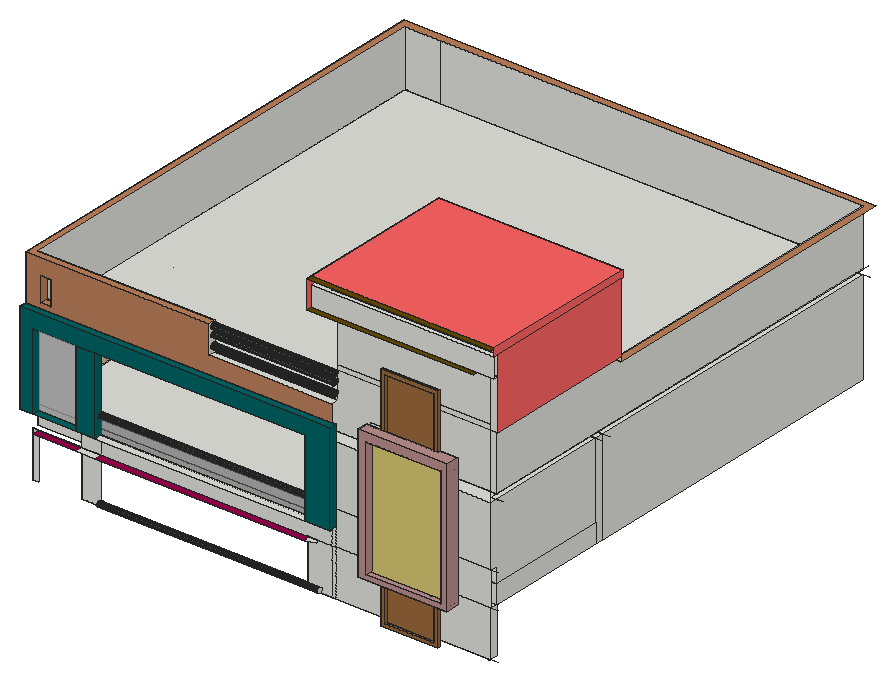
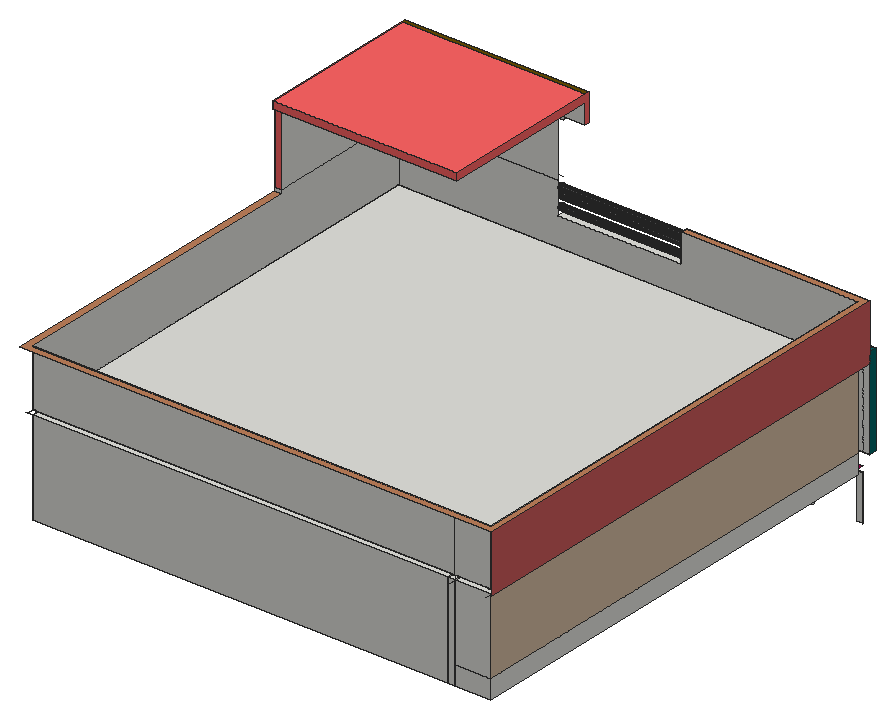
# SketchUp Ruby script. Lengths in inches.
U = 1.inch
M = Sketchup.active_model
def pt(a) = Geom::Point3d.new(a.map { |v| v * U })
def face(e, loops, mat)
  f = e.add_face(loops[0].map { |a| pt(a) })
  loops[1..].each { |l| e.add_face(l.map { |a| pt(a) }).erase! }
  f.material = f.back_material = mat if mat
  f
end
# faces: each face lists its corners as indices into pts; further lists are holes
def faces(e, pts, list, mat = nil) = list.each { |f| face(e, (f[0].is_a?(Array) ? f : [f]).map { |l| l.map { |i| pts[i] } }, mat) }
# xy, xz, yz: faces in a plane at the given z, y or x. An outline is a flat list of corners, or four numbers for a rectangle; further outlines are holes
def ring(l) = l.size == 4 ? [[l[0], l[1]], [l[2], l[1]], [l[2], l[3]], [l[0], l[3]]] : l.each_slice(2).to_a
def flat(e, list, mat, &to3) = list.each { |f| face(e, (f[0].is_a?(Array) ? f : [f]).map { |l| ring(l).map { |u, v| to3.(u, v) } }, mat) }
def xy(e, z, list, mat = nil) = flat(e, list, mat) { |x, y| [x, y, z] }
def xz(e, y, list, mat = nil) = flat(e, list, mat) { |x, z| [x, y, z] }
def yz(e, x, list, mat = nil) = flat(e, list, mat) { |y, z| [x, y, z] }
def lines(e, pts, list) = list.each { |a, b| e.add_line(pt(pts[a]), pt(pts[b])) }
# prism: a flat outline (further loops are holes) pulled along v
def prism(e, loops, v, mat = nil)
  f = face(e, loops, mat); d = Geom::Vector3d.new(v.map { |x| x * U })
  f.pushpull(f.normal.samedirection?(d) ? d.length : -d.length)
end
def box(e, o, s, mat = nil) = prism(e, [[o, [o[0] + s[0], o[1], o[2]], [o[0] + s[0], o[1] + s[1], o[2]], [o[0], o[1] + s[1], o[2]]]], [0, 0, s[2]], mat)
def at(x, y, z, deg = 0) = Geom::Transformation.translation(pt([x, y, z])) * Geom::Transformation.rotation(ORIGIN, Z_AXIS, deg.degrees)
def axes(o, x, y, z) = Geom::Transformation.new([*x, 0, *y, 0, *z, 0, *pt(o).to_a, 1])
def part(name) = M.definitions.add(name)
# library, detail: a bought-in or finely detailed component or shape, given as its bounding box
def library(name, o, s) = part(name).tap { |d| box(d.entities, o, s) }
def detail(e, o, s) = box(e.add_group.entities, o, s)
def put(e, d, t, mat = nil) = e.add_instance(d, t).tap { |i| i.material = mat if mat }
def group(e, t, mat = nil) = e.add_group.tap { |g| g.transformation = t; g.material = mat if mat }.entities
root = M.entities
M.materials.add("[0017_IndianRed]").color = [205, 92, 92]
M.materials.add("[0059_DarkOliveGreen]").color = [85, 107, 47]
M.materials.add("[0119_RosyBrown]").color = [188, 143, 143]
M.materials.add("[Color A03]").color = [255, 101, 101]
M.materials.add("[Color C04]").color = [255, 153, 50]
M.materials.add("[Color D08]").color = [102, 76, 0]
M.materials.add("[Color H08]").color = [0, 102, 102]
M.materials.add("[Color L11]").color = [153, 0, 76]
M.materials.add("[Color M05]").color = [114, 114, 114]
M.materials.add("[Color M06]").color = [86, 86, 86]
M.materials.add("[Formica Laminate Light]").color = [213, 189, 164]
M.materials.add("[Mirror 02]").color = [229, 229, 229]
M.materials.add("[Translucent Glass Gray]").color = [128, 128, 128]
M.materials["[Translucent Glass Gray]"].alpha = 0.5
M.materials.add("[Translucent Resin Crush Gray]").color = [184, 184, 184]
M.materials["[Translucent Resin Crush Gray]"].alpha = 0.8
M.materials.add("[Wood Bamboo]").color = [177, 105, 43]
M.materials.add("[Wood Board Cork]").color = [215, 201, 115]
M.materials.add("[Wood Floor]").color = [155, 105, 61]
M.materials.add("[Wood Veneer 02]").color = [190, 128, 91]
xy(root,177.05,[[623.84,156.04,695.78,159.04]],"[Wood Floor]")
xy(root,181.3125,[[236.6,165.04,523.3,165.04,523.75,165.23,236.6875,165.23],[523.3,165.04,756.04,165.04,756.04,165.23,523.75,165.23]])
xy(root,181.49,[[628.28,156.04,691.34,159.04]],"[Wood Floor]")
xy(root,182.0625,[[236.6875,165.23,756.04,165.23,756.04,174.04,241.08,174.04]])
xy(root,204,[[441.07,324.28,448.45,324.28,448.45,328.59,466.45,328.59,466.45,331.59,430.45,331.59,430.45,328.59,441.07,328.59]])
xy(root,212.33,[[533.78,326.59,672.97,328.59],[533.78,328.59,672.97,331.59]])
xy(root,215.33,[[530.78,328.59,675.97,331.59]])
xy(root,232.57,[[605.59,142.54,605.59,156.04,695.78,156.04,695.78,159.04,718.71,159.04,718.71,142.54]],"[0119_RosyBrown]")
xy(root,237.91,[[614.97,150.6,615.87,153.04],[615.87,150.6,628.28,153.04],[628.28,150.6,691.34,153.04],[691.34,150.6,695.78,153.04],[695.78,150.6,710.3125,153.04],
  [614.97,153.04,615.87,156.04],[615.87,153.04,628.28,156.04],[628.28,153.04,691.34,156.04],[691.34,153.04,695.78,156.04],[695.78,153.04,710.3125,156.04],
  [628.28,156.04,691.34,159.04],[695.78,156.04,710.3125,159.04],[616.375,159.04,623.84,159.85]])
xy(root,237.91,[[615.87,142.54,710.3125,150.6]],"[0119_RosyBrown]")
xy(root,240,[[236.6,156.04,260.92,165.04],[527.08,156.04,538.15,160.69,536.32,165.04,523.3,165.04],[174.04,165.04,174.04,165.23,236.6875,165.23,241.08,174.04,756.04,174.04,756.04,165.04,536.32,165.04,534.36,169.69,523.3,165.04],[523.3,165.04,534.36,169.69,536.32,165.04],[174.04,174.04,185.29,756.04],
  [185.29,174.04,185.29,756.04,219.49,756.04,219.49,331.59,295.38,331.59,295.38,328.59,311.1,328.59,311.1,325.59,331.38,325.59,331.38,331.59,756.04,331.59,756.04,174.04],[311.1,325.59,331.38,328.59],[295.38,328.59,331.38,331.59],[219.49,331.59,219.49,756.04,229.13,756.04,229.13,342.77,756.04,342.77,756.04,331.59],[229.13,342.77,756.04,756.04]])
xy(root,240,[[181.38,156.04,236.6,165.04],[260.92,156.04,260.92,165.04,523.3,165.04,527.08,156.04]],"[Color L11]")
xy(root,242.39,[[313.49,325.59,328.99,328.59]])
xy(root,246.83,[[355.12,328.59,402.92,331.59]])
xy(root,252.33,[[360.61,328.59,397.43,331.59]])
xy(root,255.01,[[467.84,328.59,560.59,331.59]])
xy(root,260.13,[[472.97,328.59,555.47,331.59]])
xy(root,262.875,[[165.04,156.04,174.04,165.04],[174.04,156.04,181.38,165.04],[236.6,156.04,260.92,158.48],[260.92,156.04,527.08,165.04],[527.08,156.04,558.79,165.04],
  [558.79,156.04,559.05,165.04],[236.6,158.48,260.92,160.54]])
xy(root,262.875,[[181.38,156.04,236.6,165.04]],"[Color H08]")
xy(root,263.8125,[[174.04,174.04,756.04,174.04,756.04,331.59,331.38,331.59,331.38,325.59,311.1,325.59,311.1,328.59,295.38,328.59,295.38,331.59,219.49,331.59,219.49,756.04,174.04,756.04]])
xy(root,279.61,[[313.49,325.59,328.99,328.59]],"[Wood Bamboo]")
xy(root,282,[[311.1,325.59,331.38,328.59]],"[Wood Bamboo]")
xy(root,283.3125,[[236.6,165.04,756.04,165.04,756.04,174.04,246.18,174.04]])
xy(root,323.58,[[360.61,328.59,397.43,331.59]])
xy(root,324,[[295.38,328.59,331.38,331.59]],"[Wood Bamboo]")
xy(root,327.13,[[472.97,328.59,555.47,331.59]])
xy(root,329.08,[[355.12,328.59,402.92,331.59]])
xy(root,332.25,[[467.84,328.59,560.59,331.59]])
xy(root,360,[[236.6,156.04,260.92,160.54],[236.6,160.54,260.92,165.04],[236.6,165.04,246.18,174.04,174.04,174.04,174.04,756.04,219.49,756.04,219.49,331.59,756.04,331.59,756.04,165.04],[219.49,331.59,219.49,756.04,229.13,756.04,229.13,342.77,756.04,342.77,756.04,331.59],[229.13,342.77,756.04,756.04]])
xy(root,360,[[181.38,156.04,236.6,165.04],[260.92,156.04,527.08,165.04]],"[Color H08]")
xy(root,365.75,[[755.73,174.04,756.04,756.04]])
xy(root,366,[[174.04,174.04,756.04,756.04]])
xy(root,379.73,[[165.04,156.04,558.79,165.04]],"[Color H08]")
xy(root,386.57,[[184.31,165.04,197.75,174.04]],"[Wood Veneer 02]")
xy(root,389.91,[[605.43,142.54,605.59,152.54],[614.97,150.6,615.87,152.54],[615.87,150.6,628.28,152.54],[628.28,150.6,691.34,152.54],[691.34,150.6,695.78,152.54],
  [695.78,150.6,710.3125,152.54],[605.43,152.54,605.59,153.04],[605.59,152.54,607.89,153.04],[614.97,152.54,615.87,153.04],[615.87,152.54,628.28,152.54,628.28,156.04,614.97,156.04,614.97,153.04,615.87,153.04],
  [628.28,152.54,691.34,156.04],[691.34,152.54,695.78,156.04],[695.78,152.54,710.3125,156.04],[628.28,156.04,691.34,159.04],[695.78,156.04,710.3125,159.04],
  [616.375,159.04,623.84,159.85]])
xy(root,389.91,[[615.87,142.54,710.3125,150.6]],"[0119_RosyBrown]")
xy(root,400.38,[[605.43,142.54,718.71,142.54,718.71,159.04,695.78,159.04,695.78,156.04,605.59,156.04,605.59,153.04,605.43,153.04]],"[0119_RosyBrown]")
xy(root,401.875,[[398.38,165.04,554.6,174.04]])
xy(root,417.76,[[184.31,165.04,197.75,174.04]])
xy(root,437.75,[[165.04,165.04,398.38,165.04,398.38,174.04,174.04,174.04,174.04,756.04,756.04,756.04,756.04,360.73,765.04,360.73,765.04,765.04,165.04,765.04]],"[Wood Veneer 02]")
xy(root,464.8,[[628.28,156.04,691.34,159.04]])
xy(root,469.24,[[623.84,156.04,695.78,159.04]],"[Wood Floor]")
xy(root,506.1875,[[554.6,159.04,755.73,165.04],[755.73,159.04,765.04,165.04]])
xy(root,506.1875,[[531.67,153.04,743.6,159.04]],"[Color D08]")
xy(root,531.66,[[531.67,159.04,765.04,362.6]])
xy(root,541.25,[[531.67,159.04,765.04,362.6]],"[Color A03]")
xy(root,541.25,[[531.67,153.04,765.04,159.04]],"[Color D08]")
xz(root,142.54,[[[605.59,232.57,718.71,232.57,718.71,400.38,605.43,400.38,605.43,389.91,605.59,389.91],[615.87,237.91,710.3125,389.91]]],"[0119_RosyBrown]")
xz(root,150.6,[[614.97,237.91,710.3125,389.91]],"[Wood Board Cork]")
xz(root,153.04,[[605.43,389.91,605.59,400.38]])
xz(root,156.04,[[605.59,232.57,606.34,400.38],[606.34,232.57,606.34,400.38,607.89,400.38,607.89,389.91,607.9,389.91,607.9,232.57],[607.9,232.57,607.9,389.91,614.97,389.91,614.97,237.91,623.84,237.91,623.84,232.57],[623.84,232.57,628.28,237.91],[628.28,232.57,691.34,237.91],
  [614.97,237.91,615.87,389.91],[615.87,237.91,623.84,389.91],[623.84,237.91,628.28,389.91],[691.34,237.91,695.78,389.91],[695.78,237.91,710.3125,389.91],
  [607.89,389.91,607.9,400.38],[607.9,389.91,615.87,400.38],[615.87,389.91,623.84,400.38],[623.84,389.91,628.28,400.38],[628.28,389.91,691.34,400.38],
  [691.34,389.91,695.78,400.38]])
xz(root,156.04,[[165.04,262.875,181.38,262.875,181.38,360,527.08,360,527.08,262.875,558.79,262.875,558.79,379.73,165.04,379.73],[236.6,262.875,260.92,360]],"[Color H08]")
xz(root,156.04,[[623.84,177.05,695.78,177.05,695.78,232.57,691.34,232.57,691.34,181.49,628.28,181.49,628.28,232.57,623.84,232.57],[623.84,400.38,628.28,400.38,628.28,464.8,691.34,464.8,691.34,400.38,695.78,400.38,695.78,469.24,623.84,469.24]],"[Wood Floor]")
xz(root,159.04,[[623.84,177.05,623.84,232.57,628.28,232.57,628.28,181.49,691.34,181.49,691.34,232.57,695.78,232.57,695.78,177.05],[623.84,232.57,628.28,237.91],[691.34,232.57,695.78,237.91],[695.78,232.57,695.78,237.91,710.3125,237.91,710.3125,389.91,695.78,389.91,695.78,400.38,718.71,400.38,718.71,232.57],[616.375,237.91,623.84,389.91],
  [623.84,237.91,628.28,389.91],[628.28,237.91,691.34,389.91],[691.34,237.91,695.78,389.91],[695.78,237.91,710.3125,389.91],[623.84,389.91,628.28,400.38],
  [691.34,389.91,695.78,400.38],[623.84,400.38,623.84,469.24,695.78,469.24,695.78,400.38,691.34,400.38,691.34,464.8,628.28,464.8,628.28,400.38],[531.67,506.1875,765.04,531.66]])
xz(root,159.04,[[628.28,181.49,691.34,237.91],[628.28,389.91,691.34,464.8]],"[Wood Floor]")
xz(root,159.85,[[607.89,232.57,607.89,400.38,623.84,400.38,623.84,389.91,616.375,389.91,616.375,237.91,623.84,237.91,623.84,232.57]])
xz(root,165.04,[[174.04,181.3125,181.38,240],[236.6,181.3125,260.92,240],[523.3,181.3125,554.6,240],[554.6,181.3125,559.05,240],[559.05,181.3125,755.73,240],
  [755.73,181.3125,756.04,240],[236.6,240,260.92,262.875],[260.92,240,554.6,262.875],[554.6,240,559.05,262.875],[559.05,240,559.05,262.875,558.79,262.875,558.79,283.3125,755.73,283.3125,755.73,240],
  [165.04,262.875,165.04,379.73,554.6,379.73,554.6,360,174.04,360,174.04,262.875],[174.04,262.875,181.38,360],[236.6,262.875,260.92,283.3125],[527.08,262.875,554.6,283.3125],[554.6,262.875,558.79,283.3125],
  [236.6,283.3125,260.92,360],[527.08,283.3125,527.08,284.67,537.23,284.67,537.23,288.35,527.08,288.35,527.08,360,554.6,360,554.6,283.3125],[554.6,283.3125,558.79,360],[558.79,283.3125,755.73,360],[755.73,283.3125,756.04,360],
  [260.92,284.67,527.08,288.35],[527.08,284.67,537.23,288.35],[554.6,360,558.79,379.73],[755.73,442.375,765.04,506.1875],[554.6,506.1875,755.73,531],
  [755.73,506.1875,765.04,531],[554.6,531,755.73,533.3125],[755.73,531,765.04,533.3125]])
xz(root,165.04,[[260.92,262.875,527.08,283.3125]],"[Translucent Glass Gray]")
xz(root,165.04,[[181.38,262.875,236.6,360]],"[Translucent Resin Crush Gray]")
xz(root,165.04,[[[165.04,379.73,554.6,379.73,554.6,401.875,398.38,401.875,398.38,437.75,165.04,437.75],[184.31,386.57,197.75,417.76]]],"[Wood Veneer 02]")
xz(root,165.23,[[236.6875,181.3125,523.75,182.0625],[523.75,181.3125,756.04,182.0625]])
xz(root,174.04,[[174.04,240,756.04,263.8125],[174.04,365.75,756.04,366],[[174.04,366,174.04,437.75,398.38,437.75,398.38,401.875,554.6,401.875,554.6,442.375,756.04,442.375,756.04,366],[184.31,386.57,197.75,417.76]],[554.6,442.375,756.04,531],[554.6,531,756.04,533.3125]])
xz(root,174.04,[[174.04,263.8125,174.04,360,246.18,360,246.18,283.3125,756.04,283.3125,756.04,263.8125]],"[Mirror 02]")
xz(root,325.59,[[311.1,240,331.38,240,331.38,263.8125,328.99,263.8125,328.99,242.39,313.49,242.39,313.49,263.8125,311.1,263.8125],[313.49,242.39,328.99,263.8125]])
xz(root,325.59,[[311.1,263.8125,313.49,263.8125,313.49,279.61,328.99,279.61,328.99,263.8125,331.38,263.8125,331.38,282,311.1,282]],"[Wood Bamboo]")
xz(root,328.59,[[295.38,240,311.1,263.8125],[[311.1,240,331.38,282],[313.49,242.39,328.99,279.61]]])
xz(root,328.59,[[[355.12,246.83,402.92,329.08],[360.61,252.33,397.43,323.58]],[[467.84,255.01,560.59,332.25],[472.97,260.13,555.47,327.13]]],"[Color C04]")
xz(root,328.59,[[313.49,242.39,328.99,279.61],[[295.38,263.8125,311.1,263.8125,311.1,282,331.38,282,331.38,324,295.38,324],[308.81,285.54,301.94,285.86,298.78,291.97,302.49,297.76,309.36,297.4375,312.52,291.33]],[308.81,285.54,312.52,291.33,309.36,297.4375,302.49,297.76,298.78,291.97,301.94,285.86]],"[Wood Bamboo]")
xz(root,331.59,[[219.49,240,295.38,263.8125],[295.38,240,331.38,324],[331.38,240,331.38,263.8125,355.12,263.8125,355.12,246.83,402.92,246.83,402.92,263.8125,467.84,263.8125,467.84,255.01,560.59,255.01,560.59,263.8125,756.04,263.8125,756.04,240],[355.12,246.83,355.12,263.8125,360.61,263.8125,360.61,252.33,397.43,252.33,397.43,263.8125,402.92,263.8125,402.92,246.83],[360.61,252.33,397.43,263.8125],
  [467.84,255.01,467.84,263.8125,472.97,263.8125,472.97,260.13,555.47,260.13,555.47,263.8125,560.59,263.8125,560.59,255.01],[472.97,260.13,555.47,263.8125],[355.12,263.8125,355.12,329.08,402.92,329.08,402.92,263.8125,397.43,263.8125,397.43,323.58,360.61,323.58,360.61,263.8125],[467.84,263.8125,467.84,332.25,560.59,332.25,560.59,263.8125,555.47,263.8125,555.47,327.13,472.97,327.13,472.97,263.8125]])
xz(root,331.59,[[219.49,263.8125,295.38,263.8125,295.38,324,331.38,324,331.38,263.8125,355.12,263.8125,355.12,329.08,402.92,329.08,402.92,263.8125,467.84,263.8125,467.84,332.25,560.59,332.25,560.59,263.8125,756.04,263.8125,756.04,360,219.49,360]],"[Formica Laminate Light]")
xz(root,331.59,[[360.61,263.8125,397.43,323.58],[472.97,263.8125,555.47,327.13]],"[Mirror 02]")
xz(root,342.77,[[229.13,240,621.625,360],[621.625,240,756.04,360]])
xz(root,360.73,[[756.04,437.75,765.04,442.375]])
xz(root,360.73,[[756.04,442.375,765.04,533.3125]],"[Color A03]")
xz(root,362.6,[[531.67,531.66,765.04,541.25]],"[Color A03]")
xz(root,756.04,[[174.04,240,219.49,263.8125],[219.49,240,229.13,360],[229.13,240,756.04,360],[174.04,263.8125,219.49,360],[174.04,365.75,219.49,366],
  [219.49,365.75,756.04,366],[174.04,366,219.49,437.75],[219.49,366,756.04,437.75]])
yz(root,165.04,[[165.04,365.75,765.04,437.75]],"[0017_IndianRed]")
yz(root,165.04,[[156.04,262.875,165.04,379.73]],"[Color H08]")
yz(root,174.04,[[165.04,181.3125,165.23,240],[174.04,240,756.04,263.8125],[174.04,365.75,756.04,366],[174.04,366,756.04,437.75]])
yz(root,174.04,[[174.04,263.8125,756.04,360]],"[Formica Laminate Light]")
yz(root,181.38,[[156.04,262.875,165.04,360]],"[Color H08]")
yz(root,184.31,[[165.04,386.57,174.04,417.76]],"[Wood Veneer 02]")
yz(root,197.75,[[165.04,386.57,174.04,417.76]],"[Wood Veneer 02]")
yz(root,219.49,[[331.59,240,756.04,263.8125],[331.59,263.8125,756.04,360]])
yz(root,229.13,[[342.77,240,756.04,360]])
yz(root,236.6,[[156.04,262.875,165.04,360]],"[Color H08]")
yz(root,260.92,[[165.04,284.67,165.3,285.01,165.6,285.73,165.7,286.51,165.6,287.29,165.3,288.01,165.04,288.35]])
yz(root,260.92,[[156.04,262.875,165.04,262.875,165.04,284.67,164.83,284.39,164.2,283.91,163.48,283.61,162.7,283.51,161.93,283.61,161.2,283.91,160.58,284.39,160.11,285.01,159.81,285.73,159.7,286.51,159.81,287.29,160.11,288.01,160.58,288.63,161.2,289.11,161.93,289.41,162.7,289.51,163.48,289.41,164.2,289.11,164.83,288.63,165.04,288.35,165.04,360,156.04,360]],"[Color H08]")
yz(root,295.38,[[328.59,240,331.59,263.8125]])
yz(root,295.38,[[328.59,263.8125,331.59,324]],"[Wood Bamboo]")
yz(root,311.1,[[325.59,240,328.59,263.8125]])
yz(root,311.1,[[325.59,263.8125,328.59,282]],"[Wood Bamboo]")
yz(root,313.49,[[325.59,242.39,328.59,279.61]],"[Wood Bamboo]")
yz(root,328.99,[[325.59,242.39,328.59,279.61]],"[Wood Bamboo]")
yz(root,331.38,[[325.59,240,328.59,263.8125],[328.59,240,331.59,263.8125]])
yz(root,331.38,[[325.59,263.8125,328.59,282],[328.59,263.8125,331.59,324]],"[Wood Bamboo]")
yz(root,355.12,[[328.59,246.83,331.59,329.08]],"[Color C04]")
yz(root,360.61,[[328.59,252.33,331.59,323.58]],"[Color C04]")
yz(root,397.43,[[328.59,252.33,331.59,323.58]],"[Color C04]")
yz(root,398.38,[[[165.04,401.875,174.04,437.75],[170.29,430.24,169.35,430.36,168.48,430.73,167.73,431.3,167.15,432.05,166.79,432.93,166.67,433.87,166.79,434.8,167.15,435.68,167.73,436.43,168.48,437.01,169.35,437.37,170.29,437.49,171.23,437.37,172.11,437.01,172.86,436.43,173.43,435.68,173.79,434.8,173.92,433.87,173.79,432.93,173.43,432.05,172.86,431.3,172.11,430.73,171.23,430.36],[170.29,420.3,169.35,420.43,168.48,420.79,167.73,421.37,167.15,422.12,166.79,422.99,166.67,423.93,166.79,424.87,167.15,425.74,167.73,426.49,168.48,427.07,169.35,427.43,170.29,427.55,171.23,427.43,172.11,427.07,172.86,426.49,173.43,425.74,173.79,424.87,173.92,423.93,173.79,422.99,173.43,422.12,172.86,421.37,172.11,420.79,171.23,420.43],[170.29,407.24,169.35,407.36,168.48,407.73,167.73,408.3,167.15,409.05,166.79,409.93,166.67,410.87,166.79,411.8,167.15,412.68,167.73,413.43,168.48,414.01,169.35,414.37,170.29,414.49,171.23,414.37,172.11,414.01,172.86,413.43,173.43,412.68,173.79,411.8,173.92,410.87,173.79,409.93,173.43,409.05,172.86,408.3,172.11,407.73,171.23,407.36]]])
yz(root,402.92,[[328.59,246.83,331.59,329.08]],"[Color C04]")
yz(root,467.84,[[328.59,255.01,331.59,332.25]])
yz(root,472.97,[[328.59,260.13,331.59,327.13]],"[Color C04]")
yz(root,527.08,[[156.04,262.875,165.04,360]],"[Color H08]")
yz(root,531.67,[[153.04,506.1875,153.04,541.25,362.6,541.25,362.6,531.66,159.04,531.66,159.04,506.1875]],"[Color A03]")
yz(root,537.23,[[162.7,283.51,163.48,283.61,164.2,283.91,164.83,284.39,165.04,284.67,165.04,288.35,164.83,288.63,164.2,289.11,163.48,289.41,162.7,289.51,161.93,289.41,161.2,289.11,160.58,288.63,160.11,288.01,159.81,287.29,159.7,286.51,159.81,285.73,160.11,285.01,160.58,284.39,161.2,283.91,161.93,283.61]])
yz(root,541.54,[[161.8,182.97,162.61,183.08,163.37,183.39,164.01,183.89,164.51,184.54,164.82,185.29,164.93,186.1,164.82,186.91,164.51,187.66,164.01,188.31,163.37,188.8,162.61,189.12,161.8,189.22,161,189.12,160.24,188.8,159.6,188.31,159.1,187.66,158.79,186.91,158.68,186.1,158.79,185.29,159.1,184.54,159.6,183.89,160.24,183.39,161,183.08]])
yz(root,554.6,[[165.04,531,174.04,533.3125]])
yz(root,555.47,[[328.59,260.13,331.59,327.13]],"[Color C04]")
yz(root,558.79,[[156.04,262.875,165.04,379.73]],"[Color H08]")
yz(root,560.59,[[328.59,255.01,331.59,332.25]])
yz(root,605.43,[[142.54,389.91,153.04,400.38]],"[0119_RosyBrown]")
yz(root,605.59,[[142.54,232.57,142.54,389.91,153.04,389.91,153.04,400.38,156.04,400.38,156.04,232.57]],"[0119_RosyBrown]")
yz(root,614.97,[[150.6,237.91,156.04,389.91]])
yz(root,615.87,[[142.54,237.91,153.04,389.91]],"[0119_RosyBrown]")
yz(root,616.375,[[159.04,237.91,159.85,389.91]])
yz(root,623.84,[[159.04,232.57,159.85,237.91],[159.04,389.91,159.85,400.38]])
yz(root,623.84,[[156.04,177.05,159.04,469.24]],"[Wood Floor]")
yz(root,628.28,[[156.04,237.91,159.04,389.91]])
yz(root,628.28,[[156.04,181.49,159.04,237.91],[156.04,389.91,159.04,464.8]],"[Wood Floor]")
yz(root,691.34,[[156.04,237.91,159.04,389.91]])
yz(root,691.34,[[156.04,389.91,159.04,464.8]],"[0059_DarkOliveGreen]")
yz(root,691.34,[[156.04,181.49,159.04,237.91]],"[Wood Floor]")
yz(root,695.78,[[156.04,237.91,159.04,389.91],[156.04,389.91,159.04,400.38]])
yz(root,695.78,[[156.04,177.05,159.04,232.57],[156.04,400.38,159.04,469.24]],"[Wood Floor]")
yz(root,710.3125,[[150.6,237.91,153.04,389.91],[153.04,237.91,156.04,389.91],[156.04,237.91,159.04,389.91]])
yz(root,710.3125,[[142.54,237.91,150.6,389.91]],"[0119_RosyBrown]")
yz(root,718.71,[[142.54,232.57,159.04,400.38]],"[0119_RosyBrown]")
yz(root,756.04,[[165.04,181.3125,165.04,240,174.04,240,174.04,182.0625,165.23,182.0625,165.23,181.3125],[174.04,240,331.59,263.8125],[331.59,240,342.77,360],[342.77,240,756.04,360],[174.04,263.8125,174.04,283.3125,165.04,283.3125,165.04,360,331.59,360,331.59,263.8125],
  [174.04,365.75,756.04,366],[174.04,366,174.04,442.375,360.73,442.375,360.73,437.75,756.04,437.75,756.04,366],[174.04,442.375,360.73,531],[174.04,531,360.73,533.3125]])
yz(root,765.04,[[165.04,442.375,360.73,531.66],[159.04,531.66,362.6,541.25]],"[Color A03]")
p = [[523.3,165.04,181.3125],[523.3,165.04,240],[534.36,169.69,240],[534.36,169.69,181.3125],[523.75,165.23,181.3125],[236.6875,165.23,240],
  [236.6875,165.23,182.0625],[241.08,174.04,182.0625],[241.08,174.04,240],[260.92,161,183.08],[260.92,161.8,182.97],[541.54,161.8,182.97],
  [541.54,161,183.08],[260.92,162.61,183.08],[541.54,162.61,183.08],[260.92,160.24,183.39],[541.54,160.24,183.39],[260.92,163.37,183.39],
  [541.54,163.37,183.39],[260.92,159.6,183.89],[541.54,159.6,183.89],[260.92,164.01,183.89],[541.54,164.01,183.89],[260.92,159.1,184.54],
  [541.54,159.1,184.54],[260.92,164.51,184.54],[541.54,164.51,184.54],[260.92,158.79,185.29],[541.54,158.79,185.29],[260.92,164.82,185.29],
  [541.54,164.82,185.29],[260.92,158.68,186.1],[541.54,158.68,186.1],[260.92,164.93,186.1],[541.54,164.93,186.1],[260.92,158.79,186.91],
  [541.54,158.79,186.91],[260.92,164.82,186.91],[541.54,164.82,186.91],[260.92,159.1,187.66],[541.54,159.1,187.66],[260.92,164.51,187.66],
  [541.54,164.51,187.66],[260.92,159.6,188.31],[541.54,159.6,188.31],[260.92,164.01,188.31],[541.54,164.01,188.31],[260.92,160.24,188.8],
  [541.54,160.24,188.8],[260.92,163.37,188.8],[541.54,163.37,188.8],[260.92,161,189.12],[541.54,161,189.12],[260.92,162.61,189.12],
  [541.54,162.61,189.12],[260.92,161.8,189.22],[541.54,161.8,189.22],[236.6,165.04,283.3125],[246.18,174.04,283.3125],[246.18,174.04,360],
  [236.6,165.04,360],[260.92,161.93,283.61],[260.92,162.7,283.51],[537.23,162.7,283.51],[537.23,161.93,283.61],[260.92,163.48,283.61],
  [537.23,163.48,283.61],[260.92,161.2,283.91],[537.23,161.2,283.91],[260.92,164.2,283.91],[537.23,164.2,283.91],[260.92,160.58,284.39],
  [537.23,160.58,284.39],[260.92,164.83,284.39],[537.23,164.83,284.39],[260.92,160.11,285.01],[537.23,160.11,285.01],[260.92,165.04,284.67],
  [527.08,165.04,284.67],[537.23,165.04,284.67],[260.92,159.81,285.73],[537.23,159.81,285.73],[260.92,159.7,286.51],[537.23,159.7,286.51],
  [260.92,159.81,287.29],[537.23,159.81,287.29],[260.92,160.11,288.01],[537.23,160.11,288.01],[260.92,160.58,288.63],[537.23,160.58,288.63],
  [260.92,165.04,288.35],[260.92,164.83,288.63],[537.23,164.83,288.63],[537.23,165.04,288.35],[527.08,165.04,288.35],[260.92,161.2,289.11],
  [537.23,161.2,289.11],[260.92,164.2,289.11],[537.23,164.2,289.11],[260.92,161.93,289.41],[537.23,161.93,289.41],[260.92,163.48,289.41],
  [537.23,163.48,289.41],[260.92,162.7,289.51],[537.23,162.7,289.51],[398.38,169.35,407.36],[398.38,170.29,407.24],[554.6,170.29,407.24],
  [554.6,169.35,407.36],[398.38,171.23,407.36],[554.6,171.23,407.36],[398.38,168.48,407.73],[554.6,168.48,407.73],[398.38,172.11,407.73],
  [554.6,172.11,407.73],[398.38,167.73,408.3],[554.6,167.73,408.3],[398.38,172.86,408.3],[554.6,172.86,408.3],[398.38,167.15,409.05],
  [554.6,167.15,409.05],[398.38,173.43,409.05],[554.6,173.43,409.05],[398.38,166.79,409.93],[554.6,166.79,409.93],[398.38,173.79,409.93],
  [554.6,173.79,409.93],[398.38,166.67,410.87],[554.6,166.67,410.87],[398.38,173.92,410.87],[554.6,173.92,410.87],[398.38,166.79,411.8],
  [554.6,166.79,411.8],[398.38,173.79,411.8],[554.6,173.79,411.8],[398.38,167.15,412.68],[554.6,167.15,412.68],[398.38,173.43,412.68],
  [554.6,173.43,412.68],[398.38,167.73,413.43],[554.6,167.73,413.43],[398.38,172.86,413.43],[554.6,172.86,413.43],[398.38,168.48,414.01],
  [554.6,168.48,414.01],[398.38,172.11,414.01],[554.6,172.11,414.01],[398.38,169.35,414.37],[554.6,169.35,414.37],[398.38,171.23,414.37],
  [554.6,171.23,414.37],[398.38,170.29,414.49],[554.6,170.29,414.49],[398.38,169.35,420.43],[398.38,170.29,420.3],[554.6,170.29,420.3],
  [554.6,169.35,420.43],[398.38,171.23,420.43],[554.6,171.23,420.43],[398.38,168.48,420.79],[554.6,168.48,420.79],[398.38,172.11,420.79],
  [554.6,172.11,420.79],[398.38,167.73,421.37],[554.6,167.73,421.37],[398.38,172.86,421.37],[554.6,172.86,421.37],[398.38,167.15,422.12],
  [554.6,167.15,422.12],[398.38,173.43,422.12],[554.6,173.43,422.12],[398.38,166.79,422.99],[554.6,166.79,422.99],[398.38,173.79,422.99],
  [554.6,173.79,422.99],[398.38,166.67,423.93],[554.6,166.67,423.93],[398.38,173.92,423.93],[554.6,173.92,423.93],[398.38,166.79,424.87],
  [554.6,166.79,424.87],[398.38,173.79,424.87],[554.6,173.79,424.87],[398.38,167.15,425.74],[554.6,167.15,425.74],[398.38,173.43,425.74],
  [554.6,173.43,425.74],[398.38,167.73,426.49],[554.6,167.73,426.49],[398.38,172.86,426.49],[554.6,172.86,426.49],[398.38,168.48,427.07],
  [554.6,168.48,427.07],[398.38,172.11,427.07],[554.6,172.11,427.07],[398.38,169.35,427.43],[554.6,169.35,427.43],[398.38,171.23,427.43],
  [554.6,171.23,427.43],[398.38,170.29,427.55],[554.6,170.29,427.55],[398.38,169.35,430.36],[398.38,170.29,430.24],[554.6,170.29,430.24],
  [554.6,169.35,430.36],[398.38,171.23,430.36],[554.6,171.23,430.36],[398.38,168.48,430.73],[554.6,168.48,430.73],[398.38,172.11,430.73],
  [554.6,172.11,430.73],[398.38,167.73,431.3],[554.6,167.73,431.3],[398.38,172.86,431.3],[554.6,172.86,431.3],[398.38,167.15,432.05],
  [554.6,167.15,432.05],[398.38,173.43,432.05],[554.6,173.43,432.05],[398.38,166.79,432.93],[554.6,166.79,432.93],[398.38,173.79,432.93],
  [554.6,173.79,432.93],[398.38,166.67,433.87],[554.6,166.67,433.87],[398.38,173.92,433.87],[554.6,173.92,433.87],[398.38,166.79,434.8],
  [554.6,166.79,434.8],[398.38,173.79,434.8],[554.6,173.79,434.8],[398.38,167.15,435.68],[554.6,167.15,435.68],[398.38,173.43,435.68],
  [554.6,173.43,435.68],[398.38,167.73,436.43],[554.6,167.73,436.43],[398.38,172.86,436.43],[554.6,172.86,436.43],[398.38,168.48,437.01],
  [554.6,168.48,437.01],[398.38,172.11,437.01],[554.6,172.11,437.01],[398.38,169.35,437.37],[554.6,169.35,437.37],[398.38,171.23,437.37],
  [554.6,171.23,437.37],[398.38,170.29,437.49],[554.6,170.29,437.49],[219.49,331.59,360],[219.49,331.59,366],[219.49,756.04,360],
  [219.49,756.04,365.75],[174.04,756.04,360],[174.04,765.04,360],[219.49,765.04,360],[756.04,331.59,360],[765.04,331.59,360],
  [756.04,174.04,360],[765.04,174.04,360],[756.04,342.77,360],[765.04,342.77,360],[756.04,756.04,360],[765.04,756.04,360],
  [755.73,165.04,365.75],[755.73,174.04,365.75],[755.73,756.04,365.75],[755.73,765.04,365.75],[755.73,165.04,360],[755.73,165.04,442.375],
  [765.04,165.04,365.75],[756.04,165.04,181.3125],[765.04,165.04,181.3125],[756.04,165.04,240],[765.04,165.04,240],[756.04,165.04,283.3125],
  [765.04,165.04,283.3125],[695.78,153.04,237.91],[695.78,153.04,232.57],[607.89,156.04,389.91],[607.89,153.04,389.91],[607.89,159.04,400.38],
  [607.89,159.85,400.38],[607.89,159.04,232.57],[607.89,159.85,232.57],[615.87,153.04,389.91],[615.87,153.04,400.38],[718.71,153.04,237.91],
  [710.3125,153.04,237.91],[710.3125,153.04,389.91],[718.71,153.04,389.91],[718.71,147.04,237.91],[710.3125,147.04,237.91],[554.6,165.04,442.375]]
faces(root,p,[[0,1,2,3,4]])
faces(root,p,[[5,6,7,8],[57,58,59,60]],"[Mirror 02]")
faces(root,p,[[9,10,11,12],[10,13,14,11],[15,9,12,16],[13,17,18,14],[19,15,16,20],[17,21,22,18],[23,19,20,24],[21,25,26,22],
  [27,23,24,28],[25,29,30,26],[31,27,28,32],[29,33,34,30],[35,31,32,36],[33,37,38,34],[39,35,36,40],[37,41,42,38],
  [43,39,40,44],[41,45,46,42],[47,43,44,48],[45,49,50,46],[51,47,48,52],[49,53,54,50],[55,51,52,56],[53,55,56,54],
  [61,62,63,64],[62,65,66,63],[67,61,64,68],[65,69,70,66],[71,67,68,72],[69,73,74,70],[75,71,72,76],[73,77,78,79,74],
  [80,75,76,81],[82,80,81,83],[84,82,83,85],[86,84,85,87],[88,86,87,89],[90,91,92,93,94],[95,88,89,96],[91,97,98,92],
  [99,95,96,100],[97,101,102,98],[103,99,100,104],[101,103,104,102]],"[Color M06]")
faces(root,p,[[105,106,107,108],[106,109,110,107],[111,105,108,112],[109,113,114,110],[115,111,112,116],[113,117,118,114],[119,115,116,120],[117,121,122,118],
  [123,119,120,124],[121,125,126,122],[127,123,124,128],[125,129,130,126],[131,127,128,132],[129,133,134,130],[135,131,132,136],[133,137,138,134],
  [139,135,136,140],[137,141,142,138],[143,139,140,144],[141,145,146,142],[147,143,144,148],[145,149,150,146],[151,147,148,152],[149,151,152,150],
  [153,154,155,156],[154,157,158,155],[159,153,156,160],[157,161,162,158],[163,159,160,164],[161,165,166,162],[167,163,164,168],[165,169,170,166],
  [171,167,168,172],[169,173,174,170],[175,171,172,176],[173,177,178,174],[179,175,176,180],[177,181,182,178],[183,179,180,184],[181,185,186,182],
  [187,183,184,188],[185,189,190,186],[191,187,188,192],[189,193,194,190],[195,191,192,196],[193,197,198,194],[199,195,196,200],[197,199,200,198],
  [201,202,203,204],[202,205,206,203],[207,201,204,208],[205,209,210,206],[211,207,208,212],[209,213,214,210],[215,211,212,216],[213,217,218,214],
  [219,215,216,220],[217,221,222,218],[223,219,220,224],[221,225,226,222],[227,223,224,228],[225,229,230,226],[231,227,228,232],[229,233,234,230],
  [235,231,232,236],[233,237,238,234],[239,235,236,240],[237,241,242,238],[243,239,240,244],[241,245,246,242],[247,243,244,248],[245,247,248,246]],"[Color M05]")
lines(root,p,[[249,250],[251,252],[253,254],[251,255],[256,257],[258,259],[260,261],[262,263],[264,265],[266,267],[268,264],[264,269],
  [264,270],[271,272],[273,274],[275,276],[277,278],[279,280],[281,282],[283,284],[285,286],[287,288],[289,290],[291,292],
  [269,293]])
